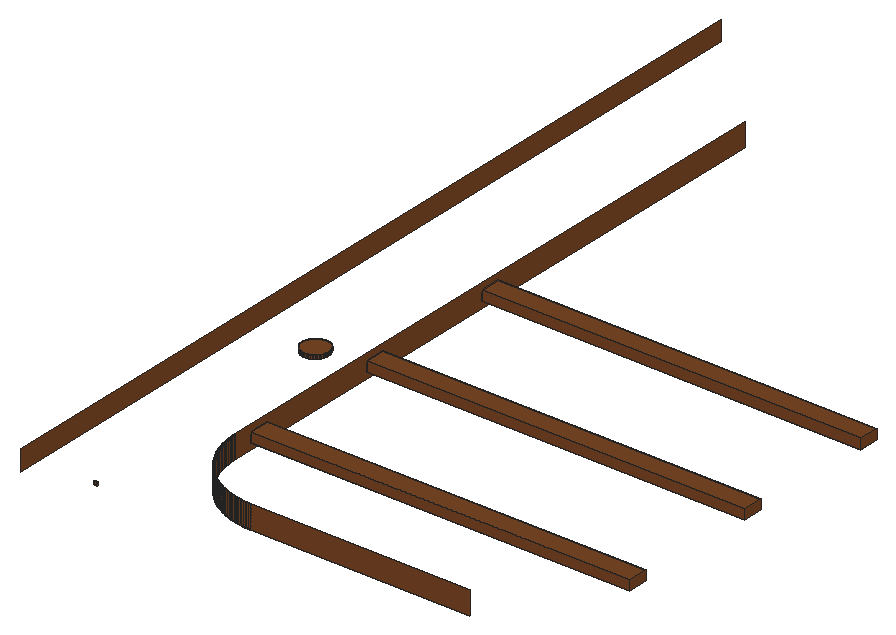
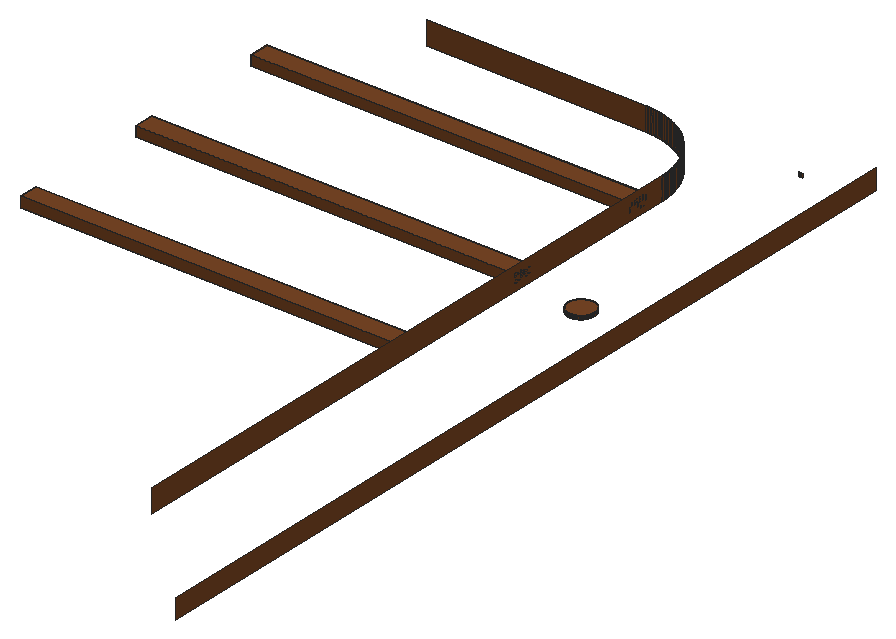
# SketchUp Ruby script. Lengths in inches.
U = 1.inch
M = Sketchup.active_model
def pt(a) = Geom::Point3d.new(a.map { |v| v * U })
def face(e, loops, mat)
  f = e.add_face(loops[0].map { |a| pt(a) })
  loops[1..].each { |l| e.add_face(l.map { |a| pt(a) }).erase! }
  f.material = f.back_material = mat if mat
  f
end
# faces: each face lists its corners as indices into pts; further lists are holes
def faces(e, pts, list, mat = nil) = list.each { |f| face(e, (f[0].is_a?(Array) ? f : [f]).map { |l| l.map { |i| pts[i] } }, mat) }
# xy, xz, yz: faces in a plane at the given z, y or x. An outline is a flat list of corners, or four numbers for a rectangle; further outlines are holes
def ring(l) = l.size == 4 ? [[l[0], l[1]], [l[2], l[1]], [l[2], l[3]], [l[0], l[3]]] : l.each_slice(2).to_a
def flat(e, list, mat, &to3) = list.each { |f| face(e, (f[0].is_a?(Array) ? f : [f]).map { |l| ring(l).map { |u, v| to3.(u, v) } }, mat) }
def xy(e, z, list, mat = nil) = flat(e, list, mat) { |x, y| [x, y, z] }
def xz(e, y, list, mat = nil) = flat(e, list, mat) { |x, z| [x, y, z] }
def yz(e, x, list, mat = nil) = flat(e, list, mat) { |y, z| [x, y, z] }
def lines(e, pts, list) = list.each { |a, b| e.add_line(pt(pts[a]), pt(pts[b])) }
# prism: a flat outline (further loops are holes) pulled along v
def prism(e, loops, v, mat = nil)
  f = face(e, loops, mat); d = Geom::Vector3d.new(v.map { |x| x * U })
  f.pushpull(f.normal.samedirection?(d) ? d.length : -d.length)
end
def box(e, o, s, mat = nil) = prism(e, [[o, [o[0] + s[0], o[1], o[2]], [o[0] + s[0], o[1] + s[1], o[2]], [o[0], o[1] + s[1], o[2]]]], [0, 0, s[2]], mat)
def at(x, y, z, deg = 0) = Geom::Transformation.translation(pt([x, y, z])) * Geom::Transformation.rotation(ORIGIN, Z_AXIS, deg.degrees)
def axes(o, x, y, z) = Geom::Transformation.new([*x, 0, *y, 0, *z, 0, *pt(o).to_a, 1])
def part(name) = M.definitions.add(name)
# library, detail: a bought-in or finely detailed component or shape, given as its bounding box
def library(name, o, s) = part(name).tap { |d| box(d.entities, o, s) }
def detail(e, o, s) = box(e.add_group.entities, o, s)
def put(e, d, t, mat = nil) = e.add_instance(d, t).tap { |i| i.material = mat if mat }
def group(e, t, mat = nil) = e.add_group.tap { |g| g.transformation = t; g.material = mat if mat }.entities
root = M.entities
M.materials.add("[Wood Veneer 01]3").color = [120, 70, 37]
c1 = part("8")
box(c1.entities,[0,0,0],[3,1.5,57],"[Wood Veneer 01]3")
xy(root,118.5,[[71.99,81.33,71.9,81.34,71.82,81.34,71.74,81.35,71.65,81.36,71.41,81.42,71.17,81.51,71.1,81.55,71.02,81.59,70.95,81.63,70.88,81.68,70.8125,81.72,70.75,81.77,70.68,81.83,70.62,81.89,70.5625,81.94,70.5,82.01,70.45,82.07,70.4,82.14,70.35,82.2,70.3,82.27,70.26,82.35,70.18,82.49,70.09,82.73,70.03,82.97,70.02,83.06,70,83.22,70,83.47,70.01,83.56,70.02,83.64,70.1,83.96,70.16,84.12,70.2,84.2,70.23,84.27,70.27,84.35,70.37,84.49,70.42,84.55,70.47,84.62,70.52,84.68,70.7,84.86,70.84,84.96,70.9,85.01,70.98,85.05,71.05,85.09,71.2,85.17,71.36,85.23,71.68,85.31,71.76,85.32,71.85,85.33,72.18,85.33,72.26,85.32,72.35,85.3,72.43,85.29,72.51,85.27,72.59,85.24,72.67,85.22,72.75,85.1875,72.83,85.15,72.9,85.12,72.98,85.08,73.05,85.04,73.12,84.99,73.1875,84.94,73.25,84.89,73.32,84.84,73.38,84.78,73.4375,84.72,73.5,84.66,73.55,84.6,73.7,84.39,73.78,84.25,73.82,84.17,73.85,84.1,73.88,84.02,73.91,83.9375,73.93,83.86,73.95,83.78,73.97,83.69,73.99,83.53,74,83.44,74,83.19,73.98,83.03,73.96,82.94,73.9,82.7,73.84,82.55,73.8,82.47,73.77,82.39,73.73,82.32,73.58,82.11,73.53,82.05,73.48,81.98,73.42,81.92,73.36,81.87,73.3,81.81,73.16,81.71,73.1,81.66,73.02,81.62,72.95,81.57,72.875,81.54,72.8,81.5,72.56,81.41,72.48,81.39,72.32,81.36,72.24,81.35,72.15,81.34,72.07,81.33]],"[Wood Veneer 01]3")
xz(root,41.99,[[71.76,118,71.85,118.5]],"[Wood Veneer 01]3")
xz(root,42,[[71.93,118,72.01,118.5],[72.01,118,72.1,118.5]],"[Wood Veneer 01]3")
xz(root,45,[[92.6875,118,92.84,121.5],[92.84,118,93,121.5],[93,118,126,121.5]],"[Wood Veneer 01]3")
xz(root,81.33,[[71.99,118,72.07,118.5]],"[Wood Veneer 01]3")
xz(root,81.34,[[71.82,118,71.9,118.5]],"[Wood Veneer 01]3")
xz(root,85.33,[[71.85,118,71.93,118.5],[71.93,118,72.01,118.5],[72.01,118,72.1,118.5],[72.1,118,72.18,118.5]],"[Wood Veneer 01]3")
yz(root,63,[[39,118,171,121]],"[Wood Veneer 01]3")
yz(root,70,[[83.22,118,83.31,118.5],[83.31,118,83.39,118.5],[83.39,118,83.47,118.5]],"[Wood Veneer 01]3")
yz(root,74,[[83.19,118,83.28,118.5],[83.28,118,83.36,118.5],[83.36,118,83.44,118.5]],"[Wood Veneer 01]3")
yz(root,81,[[56.6875,118,56.84,121.5],[56.84,118,57,121.5],[57,118,153,121.5]],"[Wood Veneer 01]3")
p = [[71.68,41.97,118],[71.76,41.99,118],[71.76,41.99,118.5],[71.68,41.97,118.5],[71.85,41.99,118],[71.93,42,118],
  [71.93,42,118.5],[71.85,41.99,118.5],[72.1,42,118],[72.18,41.99,118],[72.18,41.99,118.5],[72.1,42,118.5],
  [72.26,41.98,118],[72.26,41.98,118.5],[91.9,45.05,118],[91.9,45.05,121],[91.9,45.05,121.5],[92.06,45.04,121.5],
  [92.06,45.04,121],[92.06,45.04,118],[92.22,45.03,121.5],[92.22,45.03,121],[92.22,45.03,118],[92.37,45.02,121.5],
  [92.37,45.02,121],[92.37,45.02,118],[92.53,45.01,121.5],[92.53,45.01,121],[92.53,45.01,118],[92.6875,45,121.5],
  [92.6875,45,121],[92.6875,45,118],[90.97,45.17,118],[90.97,45.17,121],[90.97,45.17,121.5],[91.12,45.15,121.5],
  [91.12,45.15,121],[91.12,45.15,118],[91.28,45.125,121.5],[91.28,45.125,121],[91.28,45.125,118],[91.43,45.1,121.5],
  [91.43,45.1,121],[91.43,45.1,118],[91.59,45.08,121.5],[91.59,45.08,121],[91.59,45.08,118],[91.75,45.07,121.5],
  [91.75,45.07,121],[91.75,45.07,118],[90.51,45.26,118],[90.51,45.26,121],[90.51,45.26,121.5],[90.66,45.23,121.5],
  [90.66,45.23,121],[90.66,45.23,118],[90.8125,45.2,121.5],[90.8125,45.2,121],[90.8125,45.2,118],[90.05,45.37,118],
  [90.05,45.37,121],[90.05,45.37,121.5],[90.2,45.33,121.5],[90.2,45.33,121],[90.2,45.33,118],[90.35,45.3,121.5],
  [90.35,45.3,121],[90.35,45.3,118],[89.74,45.45,118],[89.74,45.45,121],[89.74,45.45,121.5],[89.89,45.41,121.5],
  [89.89,45.41,121],[89.89,45.41,118],[89.29,45.59,118],[89.29,45.59,121],[89.29,45.59,121.5],[89.44,45.54,121.5],
  [89.44,45.54,121],[89.44,45.54,118],[89.59,45.49,121.5],[89.59,45.49,121],[89.59,45.49,118],[88.99,45.6875,118],
  [88.99,45.6875,121],[88.99,45.6875,121.5],[89.14,45.64,121.5],[89.14,45.64,121],[89.14,45.64,118],[88.7,45.8,118],
  [88.7,45.8,121],[88.7,45.8,121.5],[88.85,45.74,121.5],[88.85,45.74,121],[88.85,45.74,118],[88.55,45.85,118],
  [88.55,45.85,121],[88.55,45.85,121.5],[88.26,45.97,118],[88.26,45.97,121],[88.26,45.97,121.5],[88.41,45.91,121.5],
  [88.41,45.91,121],[88.41,45.91,118],[87.98,46.1,118],[87.98,46.1,121],[87.98,46.1,121.5],[88.12,46.04,121.5],
  [88.12,46.04,121],[88.12,46.04,118],[87.83,46.17,118],[87.83,46.17,121],[87.83,46.17,121.5],[87.55,46.31,118],
  [87.55,46.31,121],[87.55,46.31,121.5],[87.69,46.24,121.5],[87.69,46.24,121],[87.69,46.24,118],[87.41,46.38,118],
  [87.41,46.38,121],[87.41,46.38,121.5],[87.27,46.45,118],[87.27,46.45,121],[87.27,46.45,121.5],[87,46.61,118],
  [87,46.61,121],[87,46.61,121.5],[87.14,46.53,121.5],[87.14,46.53,121],[87.14,46.53,118],[86.86,46.6875,118],
  [86.86,46.6875,121],[86.86,46.6875,121.5],[86.73,46.77,118],[86.73,46.77,121],[86.73,46.77,121.5],[86.6,46.85,118],
  [86.6,46.85,121],[86.6,46.85,121.5],[86.33,47.02,118],[86.33,47.02,121],[86.33,47.02,121.5],[86.46,46.9375,121.5],
  [86.46,46.9375,121],[86.46,46.9375,118],[86.2,47.11,118],[86.2,47.11,121],[86.2,47.11,121.5],[86.07,47.2,118],
  [86.07,47.2,121],[86.07,47.2,121.5],[85.95,47.29,118],[85.95,47.29,121],[85.95,47.29,121.5],[85.82,47.38,118],
  [85.82,47.38,121],[85.82,47.38,121.5],[85.69,47.48,118],[85.69,47.48,121],[85.69,47.48,121.5],[85.57,47.58,118],
  [85.57,47.58,121],[85.57,47.58,121.5],[85.45,47.67,118],[85.45,47.67,121],[85.45,47.67,121.5],[85.33,47.77,118],
  [85.33,47.77,121],[85.33,47.77,121.5],[85.21,47.875,118],[85.21,47.875,121],[85.21,47.875,121.5],[85.09,47.98,118],
  [85.09,47.98,121],[85.09,47.98,121.5],[84.97,48.08,118],[84.97,48.08,121],[84.97,48.08,121.5],[84.85,48.1875,118],
  [84.85,48.1875,121],[84.85,48.1875,121.5],[84.74,48.3,118],[84.74,48.3,121],[84.74,48.3,121.5],[84.625,48.4,118],
  [84.625,48.4,121],[84.625,48.4,121.5],[84.51,48.51,118],[84.51,48.51,121],[84.51,48.51,121.5],[84.4,48.625,118],
  [84.4,48.625,121],[84.4,48.625,121.5],[84.3,48.74,118],[84.3,48.74,121],[84.3,48.74,121.5],[84.1875,48.85,118],
  [84.1875,48.85,121],[84.1875,48.85,121.5],[84.08,48.97,118],[84.08,48.97,121],[84.08,48.97,121.5],[83.98,49.09,118],
  [83.98,49.09,121],[83.98,49.09,121.5],[83.875,49.21,118],[83.875,49.21,121],[83.875,49.21,121.5],[83.77,49.33,118],
  [83.77,49.33,121],[83.77,49.33,121.5],[83.67,49.45,118],[83.67,49.45,121],[83.67,49.45,121.5],[83.58,49.57,118],
  [83.58,49.57,121],[83.58,49.57,121.5],[83.48,49.69,118],[83.48,49.69,121],[83.48,49.69,121.5],[83.38,49.82,118],
  [83.38,49.82,121],[83.38,49.82,121.5],[83.29,49.95,118],[83.29,49.95,121],[83.29,49.95,121.5],[83.2,50.07,118],
  [83.2,50.07,121],[83.2,50.07,121.5],[83.11,50.2,118],[83.11,50.2,121],[83.11,50.2,121.5],[83.02,50.33,118],
  [83.02,50.33,121],[83.02,50.33,121.5],[82.9375,50.46,118],[82.9375,50.46,121],[82.9375,50.46,121.5],[82.85,50.6,118],
  [82.85,50.6,121],[82.85,50.6,121.5],[82.77,50.73,118],[82.77,50.73,121],[82.77,50.73,121.5],[82.6875,50.86,118],
  [82.6875,50.86,121],[82.6875,50.86,121.5],[82.61,51,118],[82.61,51,121],[82.61,51,121.5],[82.53,51.14,118],
  [82.53,51.14,121],[82.53,51.14,121.5],[82.45,51.27,118],[82.45,51.27,121],[82.45,51.27,121.5],[82.38,51.41,118],
  [82.38,51.41,121],[82.38,51.41,121.5],[82.31,51.55,118],[82.31,51.55,121],[82.31,51.55,121.5],[82.24,51.69,118],
  [82.24,51.69,121],[82.24,51.69,121.5],[82.17,51.83,118],[82.17,51.83,121],[82.17,51.83,121.5],[82.1,51.98,118],
  [82.1,51.98,121],[82.1,51.98,121.5],[82.04,52.12,118],[82.04,52.12,121],[82.04,52.12,121.5],[81.97,52.26,118],
  [81.97,52.26,121],[81.97,52.26,121.5],[81.91,52.41,118],[81.91,52.41,121],[81.91,52.41,121.5],[81.85,52.55,118],
  [81.85,52.55,121],[81.85,52.55,121.5],[81.8,52.7,118],[81.8,52.7,121],[81.8,52.7,121.5],[81.74,52.85,118],
  [81.74,52.85,121],[81.74,52.85,121.5],[81.6875,52.99,118],[81.6875,52.99,121],[81.6875,52.99,121.5],[81.64,53.14,118],
  [81.64,53.14,121],[81.64,53.14,121.5],[81.59,53.29,118],[81.59,53.29,121],[81.59,53.29,121.5],[81.54,53.44,118],
  [81.54,53.44,121],[81.54,53.44,121.5],[81.49,53.59,118],[81.49,53.59,121],[81.49,53.59,121.5],[81.45,53.74,118],
  [81.45,53.74,121],[81.45,53.74,121.5],[81.41,53.89,118],[81.41,53.89,121],[81.41,53.89,121.5],[81.37,54.05,118],
  [81.37,54.05,121],[81.37,54.05,121.5],[81.33,54.2,118],[81.33,54.2,121],[81.33,54.2,121.5],[81.3,54.35,118],
  [81.3,54.35,121],[81.3,54.35,121.5],[81.26,54.51,118],[81.26,54.51,121],[81.26,54.51,121.5],[81.23,54.66,118],
  [81.23,54.66,121],[81.23,54.66,121.5],[81.2,54.8125,118],[81.2,54.8125,121],[81.2,54.8125,121.5],[81.17,54.97,118],
  [81.17,54.97,121],[81.17,54.97,121.5],[81.15,55.12,118],[81.15,55.12,121],[81.15,55.12,121.5],[81.125,55.28,118],
  [81.125,55.28,121],[81.125,55.28,121.5],[81.1,55.43,118],[81.1,55.43,121],[81.1,55.43,121.5],[81.08,55.59,118],
  [81.08,55.59,121],[81.08,55.59,121.5],[81.07,55.75,118],[81.07,55.75,121],[81.07,55.75,121.5],[81.05,55.9,118],
  [81.05,55.9,121],[81.05,55.9,121.5],[81.04,56.06,118],[81.04,56.06,121],[81.04,56.06,121.5],[81.03,56.22,118],
  [81.03,56.22,121],[81.03,56.22,121.5],[81.02,56.37,118],[81.02,56.37,121],[81.02,56.37,121.5],[81.01,56.53,118],
  [81.01,56.53,121],[81.01,56.53,121.5],[81,56.6875,118],[81,56.6875,121],[81,56.6875,121.5],[71.82,81.34,118],
  [71.74,81.35,118],[71.74,81.35,118.5],[71.82,81.34,118.5],[71.99,81.33,118],[71.9,81.34,118],[71.9,81.34,118.5],
  [71.99,81.33,118.5],[72.15,81.34,118],[72.07,81.33,118],[72.07,81.33,118.5],[72.15,81.34,118.5],[72.24,81.35,118],
  [72.24,81.35,118.5],[72.32,81.36,118],[72.32,81.36,118.5],[71.41,81.42,118],[71.33,81.45,118],[71.33,81.45,118.5],
  [71.41,81.42,118.5],[71.25,81.48,118],[71.25,81.48,118.5],[71.49,81.4,118],[71.49,81.4,118.5],[71.57,81.38,118],
  [71.57,81.38,118.5],[71.65,81.36,118],[71.65,81.36,118.5],[72.4,81.375,118],[72.4,81.375,118.5],[72.48,81.39,118],
  [72.48,81.39,118.5],[72.56,81.41,118],[72.56,81.41,118.5],[72.64,81.44,118],[72.64,81.44,118.5],[72.72,81.47,118],
  [72.72,81.47,118.5],[71.1,81.55,118],[71.02,81.59,118],[71.02,81.59,118.5],[71.1,81.55,118.5],[71.17,81.51,118],
  [71.17,81.51,118.5],[72.8,81.5,118],[72.8,81.5,118.5],[72.875,81.54,118],[72.875,81.54,118.5],[72.95,81.57,118],
  [72.95,81.57,118.5],[70.95,81.63,118],[70.88,81.68,118],[70.88,81.68,118.5],[70.95,81.63,118.5],[73.02,81.62,118],
  [73.02,81.62,118.5],[73.1,81.66,118],[73.1,81.66,118.5],[70.8125,81.72,118],[70.75,81.77,118],[70.75,81.77,118.5],
  [70.8125,81.72,118.5],[73.16,81.71,118],[73.16,81.71,118.5],[73.23,81.76,118],[73.23,81.76,118.5],[70.68,81.83,118],
  [70.62,81.89,118],[70.62,81.89,118.5],[70.68,81.83,118.5],[73.3,81.81,118],[73.3,81.81,118.5],[73.36,81.87,118],
  [73.36,81.87,118.5],[70.5625,81.94,118],[70.5,82.01,118],[70.5,82.01,118.5],[70.5625,81.94,118.5],[73.42,81.92,118],
  [73.42,81.92,118.5],[73.48,81.98,118],[73.48,81.98,118.5],[70.45,82.07,118],[70.45,82.07,118.5],[73.53,82.05,118],
  [73.53,82.05,118.5],[73.58,82.11,118],[73.58,82.11,118.5],[70.4,82.14,118],[70.35,82.2,118],[70.35,82.2,118.5],
  [70.4,82.14,118.5],[73.63,82.18,118],[73.63,82.18,118.5],[70.3,82.27,118],[70.3,82.27,118.5],[73.68,82.25,118],
  [73.68,82.25,118.5],[73.73,82.32,118],[73.73,82.32,118.5],[70.26,82.35,118],[70.22,82.42,118],[70.22,82.42,118.5],
  [70.26,82.35,118.5],[73.77,82.39,118],[73.77,82.39,118.5],[70.18,82.49,118],[70.18,82.49,118.5],[73.8,82.47,118],
  [73.8,82.47,118.5],[70.15,82.57,118],[70.15,82.57,118.5],[73.84,82.55,118],[73.84,82.55,118.5],[73.87,82.625,118],
  [73.87,82.625,118.5],[70.12,82.65,118],[70.12,82.65,118.5],[70.09,82.73,118],[70.09,82.73,118.5],[73.9,82.7,118],
  [73.9,82.7,118.5],[70.07,82.81,118],[70.07,82.81,118.5],[73.92,82.78,118],[73.92,82.78,118.5],[70.05,82.89,118],
  [70.05,82.89,118.5],[73.94,82.86,118],[73.94,82.86,118.5],[70.03,82.97,118],[70.03,82.97,118.5],[73.96,82.94,118],
  [73.96,82.94,118.5],[73.98,83.03,118],[73.98,83.03,118.5],[70.02,83.06,118],[70.02,83.06,118.5],[73.99,83.11,118],
  [73.99,83.11,118.5],[70.01,83.14,118],[70.01,83.14,118.5],[70,83.22,118],[70,83.22,118.5],[74,83.19,118],
  [74,83.19,118.5],[73.99,83.53,118],[74,83.44,118],[74,83.44,118.5],[73.99,83.53,118.5],[70,83.47,118],
  [70.01,83.56,118],[70.01,83.56,118.5],[70,83.47,118.5],[73.98,83.61,118],[73.98,83.61,118.5],[70.02,83.64,118],
  [70.02,83.64,118.5],[70.04,83.72,118],[70.04,83.72,118.5],[73.97,83.69,118],[73.97,83.69,118.5],[70.06,83.8,118],
  [70.06,83.8,118.5],[73.95,83.78,118],[73.95,83.78,118.5],[70.08,83.88,118],[70.08,83.88,118.5],[73.93,83.86,118],
  [73.93,83.86,118.5],[70.1,83.96,118],[70.1,83.96,118.5],[73.91,83.9375,118],[73.91,83.9375,118.5],[73.88,84.02,118],
  [73.88,84.02,118.5],[70.13,84.04,118],[70.13,84.04,118.5],[70.16,84.12,118],[70.16,84.12,118.5],[73.85,84.1,118],
  [73.85,84.1,118.5],[70.2,84.2,118],[70.2,84.2,118.5],[73.82,84.17,118],[73.82,84.17,118.5],[70.23,84.27,118],
  [70.23,84.27,118.5],[73.74,84.32,118],[73.78,84.25,118],[73.78,84.25,118.5],[73.74,84.32,118.5],[70.27,84.35,118],
  [70.27,84.35,118.5],[70.32,84.42,118],[70.32,84.42,118.5],[73.7,84.39,118],[73.7,84.39,118.5],[70.37,84.49,118],
  [70.37,84.49,118.5],[73.65,84.46,118],[73.65,84.46,118.5],[70.42,84.55,118],[70.42,84.55,118.5],[73.55,84.6,118],
  [73.6,84.53,118],[73.6,84.53,118.5],[73.55,84.6,118.5],[70.47,84.62,118],[70.47,84.62,118.5],[70.52,84.68,118],
  [70.52,84.68,118.5],[73.5,84.66,118],[73.5,84.66,118.5],[70.58,84.74,118],[70.58,84.74,118.5],[70.64,84.8,118],
  [70.64,84.8,118.5],[73.4375,84.72,118],[73.4375,84.72,118.5],[73.38,84.78,118],[73.38,84.78,118.5],[70.7,84.86,118],
  [70.7,84.86,118.5],[73.32,84.84,118],[73.32,84.84,118.5],[73.25,84.89,118],[73.25,84.89,118.5],[70.77,84.91,118],
  [70.77,84.91,118.5],[70.84,84.96,118],[70.84,84.96,118.5],[73.12,84.99,118],[73.1875,84.94,118],[73.1875,84.94,118.5],
  [73.12,84.99,118.5],[70.9,85.01,118],[70.9,85.01,118.5],[70.98,85.05,118],[70.98,85.05,118.5],[73.05,85.04,118],
  [73.05,85.04,118.5],[72.98,85.08,118],[72.98,85.08,118.5],[71.05,85.09,118],[71.05,85.09,118.5],[71.125,85.13,118],
  [71.125,85.13,118.5],[71.2,85.17,118],[71.2,85.17,118.5],[72.83,85.15,118],[72.9,85.12,118],[72.9,85.12,118.5],
  [72.83,85.15,118.5],[71.28,85.2,118],[71.28,85.2,118.5],[71.36,85.23,118],[71.36,85.23,118.5],[71.44,85.25,118],
  [71.44,85.25,118.5],[72.51,85.27,118],[72.59,85.24,118],[72.59,85.24,118.5],[72.51,85.27,118.5],[72.67,85.22,118],
  [72.67,85.22,118.5],[72.75,85.1875,118],[72.75,85.1875,118.5],[71.52,85.27,118],[71.52,85.27,118.5],[71.6,85.29,118],
  [71.6,85.29,118.5],[71.68,85.31,118],[71.68,85.31,118.5],[71.76,85.32,118],[71.76,85.32,118.5],[71.85,85.33,118],
  [71.85,85.33,118.5],[72.18,85.33,118],[72.26,85.32,118],[72.26,85.32,118.5],[72.18,85.33,118.5],[72.35,85.3,118],
  [72.43,85.29,118],[72.43,85.29,118.5],[72.35,85.3,118.5]]
faces(root,p,[[0,1,2,3],[4,5,6,7],[8,9,10,11],[9,12,13,10],[14,15,16,17,18,19],[19,18,17,20,21,22],[22,21,20,23,24,25],[25,24,23,26,27,28],
  [28,27,26,29,30,31],[32,33,34,35,36,37],[37,36,35,38,39,40],[40,39,38,41,42,43],[43,42,41,44,45,46],[46,45,44,47,48,49],[49,48,47,16,15,14],[50,51,52,53,54,55],
  [55,54,53,56,57,58],[58,57,56,34,33,32],[59,60,61,62,63,64],[64,63,62,65,66,67],[67,66,65,52,51,50],[68,69,70,71,72,73],[73,72,71,61,60,59],[74,75,76,77,78,79],
  [79,78,77,80,81,82],[82,81,80,70,69,68],[83,84,85,86,87,88],[88,87,86,76,75,74],[89,90,91,92,93,94],[94,93,92,85,84,83],[95,96,97,91,90,89],[98,99,100,101,102,103],
  [103,102,101,97,96,95],[104,105,106,107,108,109],[109,108,107,100,99,98],[110,111,112,106,105,104],[113,114,115,116,117,118],[118,117,116,112,111,110],[119,120,121,115,114,113],[122,123,124,121,120,119],
  [125,126,127,128,129,130],[130,129,128,124,123,122],[131,132,133,127,126,125],[134,135,136,133,132,131],[137,138,139,136,135,134],[140,141,142,143,144,145],[145,144,143,139,138,137],[146,147,148,142,141,140],
  [149,150,151,148,147,146],[152,153,154,151,150,149],[155,156,157,154,153,152],[158,159,160,157,156,155],[161,162,163,160,159,158],[164,165,166,163,162,161],[167,168,169,166,165,164],[170,171,172,169,168,167],
  [173,174,175,172,171,170],[176,177,178,175,174,173],[179,180,181,178,177,176],[182,183,184,181,180,179],[185,186,187,184,183,182],[188,189,190,187,186,185],[191,192,193,190,189,188],[194,195,196,193,192,191],
  [197,198,199,196,195,194],[200,201,202,199,198,197],[203,204,205,202,201,200],[206,207,208,205,204,203],[209,210,211,208,207,206],[212,213,214,211,210,209],[215,216,217,214,213,212],[218,219,220,217,216,215],
  [221,222,223,220,219,218],[224,225,226,223,222,221],[227,228,229,226,225,224],[230,231,232,229,228,227],[233,234,235,232,231,230],[236,237,238,235,234,233],[239,240,241,238,237,236],[242,243,244,241,240,239],
  [245,246,247,244,243,242],[248,249,250,247,246,245],[251,252,253,250,249,248],[254,255,256,253,252,251],[257,258,259,256,255,254],[260,261,262,259,258,257],[263,264,265,262,261,260],[266,267,268,265,264,263],
  [269,270,271,268,267,266],[272,273,274,271,270,269],[275,276,277,274,273,272],[278,279,280,277,276,275],[281,282,283,280,279,278],[284,285,286,283,282,281],[287,288,289,286,285,284],[290,291,292,289,288,287],
  [293,294,295,292,291,290],[296,297,298,295,294,293],[299,300,301,298,297,296],[302,303,304,301,300,299],[305,306,307,304,303,302],[308,309,310,307,306,305],[311,312,313,310,309,308],[314,315,316,313,312,311],
  [317,318,319,316,315,314],[320,321,322,319,318,317],[323,324,325,322,321,320],[326,327,328,325,324,323],[329,330,331,328,327,326],[332,333,334,331,330,329],[335,336,337,334,333,332],[338,339,340,337,336,335],
  [341,342,343,340,339,338],[344,345,346,343,342,341],[347,348,349,346,345,344],[350,351,352,349,348,347],[353,354,355,352,351,350],[356,357,358,355,354,353],[359,360,361,358,357,356],[362,363,364,361,360,359],
  [365,366,367,368],[369,370,371,372],[373,374,375,376],[377,373,376,378],[379,377,378,380],[381,382,383,384],[382,385,386,383],[387,381,384,388],
  [389,387,388,390],[391,389,390,392],[366,391,392,367],[393,379,380,394],[395,393,394,396],[397,395,396,398],[399,397,398,400],[401,399,400,402],
  [403,404,405,406],[407,403,406,408],[385,407,408,386],[409,401,402,410],[411,409,410,412],[413,411,412,414],[415,416,417,418],[404,415,418,405],
  [419,413,414,420],[421,419,420,422],[423,424,425,426],[416,423,426,417],[427,421,422,428],[429,427,428,430],[431,432,433,434],[424,431,434,425],
  [435,429,430,436],[437,435,436,438],[439,440,441,442],[432,439,442,433],[443,437,438,444],[445,443,444,446],[440,447,448,441],[449,445,446,450],
  [451,449,450,452],[453,454,455,456],[447,453,456,448],[457,451,452,458],[454,459,460,455],[461,457,458,462],[463,461,462,464],[465,466,467,468],
  [459,465,468,460],[469,463,464,470],[466,471,472,467],[473,469,470,474],[471,475,476,472],[477,473,474,478],[479,477,478,480],[475,481,482,476],
  [481,483,484,482],[485,479,480,486],[483,487,488,484],[489,485,486,490],[487,491,492,488],[493,489,490,494],[491,495,496,492],[497,493,494,498],
  [499,497,498,500],[495,501,502,496],[503,499,500,504],[501,505,506,502],[505,507,508,506],[509,503,504,510],[511,512,513,514],[515,516,517,518],
  [519,511,514,520],[516,521,522,517],[521,523,524,522],[525,519,520,526],[523,527,528,524],[529,525,526,530],[527,531,532,528],[533,529,530,534],
  [531,535,536,532],[537,533,534,538],[539,537,538,540],[535,541,542,536],[541,543,544,542],[545,539,540,546],[543,547,548,544],[549,545,546,550],
  [547,551,552,548],[553,554,555,556],[554,549,550,555],[551,557,558,552],[557,559,560,558],[561,553,556,562],[559,563,564,560],[565,561,562,566],
  [563,567,568,564],[569,570,571,572],[570,565,566,571],[567,573,574,568],[573,575,576,574],[577,569,572,578],[575,579,580,576],[579,581,582,580],
  [583,577,578,584],[585,583,584,586],[581,587,588,582],[589,585,586,590],[591,589,590,592],[587,593,594,588],[593,595,596,594],[597,598,599,600],
  [598,591,592,599],[595,601,602,596],[601,603,604,602],[605,597,600,606],[607,605,606,608],[603,609,610,604],[609,611,612,610],[611,613,614,612],
  [615,616,617,618],[616,607,608,617],[613,619,620,614],[619,621,622,620],[621,623,624,622],[625,626,627,628],[626,629,630,627],[631,615,618,632],
  [629,631,632,630],[623,633,634,624],[633,635,636,634],[635,637,638,636],[637,639,640,638],[639,641,642,640],[643,644,645,646],[647,648,649,650],
  [644,647,650,645],[648,625,628,649]],"[Wood Veneer 01]3")
put(root,c1,axes([81,60,119],[0,1,0],[0,0,1],[1,0,0]))
put(root,c1,axes([81,81.75,119],[0,1,0],[0,0,1],[1,0,0]))
put(root,c1,axes([81,103.5,119],[0,1,0],[0,0,1],[1,0,0]))
